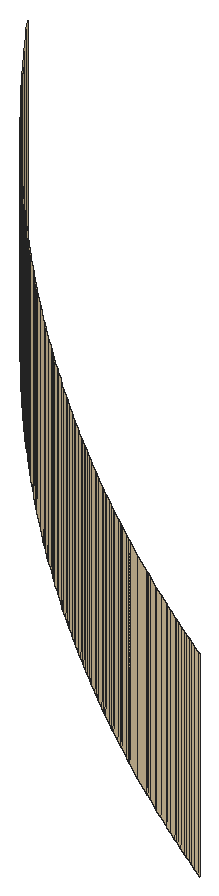
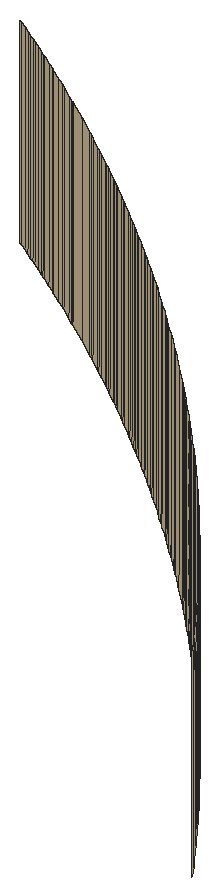
# SketchUp Ruby script. Lengths in inches.
U = 1.inch
M = Sketchup.active_model
def pt(a) = Geom::Point3d.new(a.map { |v| v * U })
def face(e, loops, mat)
  f = e.add_face(loops[0].map { |a| pt(a) })
  loops[1..].each { |l| e.add_face(l.map { |a| pt(a) }).erase! }
  f.material = f.back_material = mat if mat
  f
end
# faces: each face lists its corners as indices into pts; further lists are holes
def faces(e, pts, list, mat = nil) = list.each { |f| face(e, (f[0].is_a?(Array) ? f : [f]).map { |l| l.map { |i| pts[i] } }, mat) }
# xy, xz, yz: faces in a plane at the given z, y or x. An outline is a flat list of corners, or four numbers for a rectangle; further outlines are holes
def ring(l) = l.size == 4 ? [[l[0], l[1]], [l[2], l[1]], [l[2], l[3]], [l[0], l[3]]] : l.each_slice(2).to_a
def flat(e, list, mat, &to3) = list.each { |f| face(e, (f[0].is_a?(Array) ? f : [f]).map { |l| ring(l).map { |u, v| to3.(u, v) } }, mat) }
def xy(e, z, list, mat = nil) = flat(e, list, mat) { |x, y| [x, y, z] }
def xz(e, y, list, mat = nil) = flat(e, list, mat) { |x, z| [x, y, z] }
def yz(e, x, list, mat = nil) = flat(e, list, mat) { |y, z| [x, y, z] }
def lines(e, pts, list) = list.each { |a, b| e.add_line(pt(pts[a]), pt(pts[b])) }
# prism: a flat outline (further loops are holes) pulled along v
def prism(e, loops, v, mat = nil)
  f = face(e, loops, mat); d = Geom::Vector3d.new(v.map { |x| x * U })
  f.pushpull(f.normal.samedirection?(d) ? d.length : -d.length)
end
def box(e, o, s, mat = nil) = prism(e, [[o, [o[0] + s[0], o[1], o[2]], [o[0] + s[0], o[1] + s[1], o[2]], [o[0], o[1] + s[1], o[2]]]], [0, 0, s[2]], mat)
def at(x, y, z, deg = 0) = Geom::Transformation.translation(pt([x, y, z])) * Geom::Transformation.rotation(ORIGIN, Z_AXIS, deg.degrees)
def axes(o, x, y, z) = Geom::Transformation.new([*x, 0, *y, 0, *z, 0, *pt(o).to_a, 1])
def part(name) = M.definitions.add(name)
# library, detail: a bought-in or finely detailed component or shape, given as its bounding box
def library(name, o, s) = part(name).tap { |d| box(d.entities, o, s) }
def detail(e, o, s) = box(e.add_group.entities, o, s)
def put(e, d, t, mat = nil) = e.add_instance(d, t).tap { |i| i.material = mat if mat }
def group(e, t, mat = nil) = e.add_group.tap { |g| g.transformation = t; g.material = mat if mat }.entities
root = M.entities
M.materials.add("1026 AP 7946 SUNNY SIDE UP").color = [254, 231, 186]
p = [[16.068,217.047,276],[16.027,217.074,276],[16.027,217.074,274],[16.068,217.047,274],[15.982,217.102,276],[15.905,217.152,276],
  [15.905,217.152,274],[15.982,217.102,274],[15.768,217.241,276],[15.682,217.298,276],[15.682,217.298,274],[15.768,217.241,274],
  [15.805,217.217,276],[15.805,217.217,274],[15.839,217.195,276],[15.839,217.195,274],[15.612,217.344,276],[15.584,217.362,276],
  [15.584,217.362,274],[15.612,217.344,274],[15.46,217.446,276],[15.386,217.496,276],[15.386,217.496,274],[15.46,217.446,274],
  [15.555,217.382,276],[15.555,217.382,274],[15.344,217.525,276],[15.236,217.599,276],[15.236,217.599,274],[15.344,217.525,274],
  [15.365,217.51,276],[15.365,217.51,274],[15.161,217.65,276],[15.161,217.65,274],[15.133,217.67,276],[15.006,217.759,276],
  [15.006,217.759,274],[15.133,217.67,274],[15.148,217.66,276],[15.148,217.66,274],[14.925,217.817,276],[14.718,217.966,276],
  [14.718,217.966,274],[14.925,217.817,274],[14.932,217.812,276],[14.932,217.812,274],[14.939,217.807,276],[14.939,217.807,274],
  [14.512,218.117,276],[14.512,218.117,274],[14.498,218.127,276],[14.432,218.176,276],[14.432,218.176,274],[14.498,218.127,274],
  [14.505,218.122,276],[14.505,218.122,274],[14.308,218.27,276],[14.308,218.27,274],[14.209,218.345,276],[14.105,218.425,276],
  [14.105,218.425,274],[14.209,218.345,274],[14.28,218.29,276],[14.28,218.29,274],[14.294,218.28,276],[14.294,218.28,274],
  [14.084,218.441,276],[14.064,218.456,276],[14.064,218.456,274],[14.084,218.441,274],[13.994,218.511,276],[13.904,218.582,276],
  [13.904,218.582,274],[13.994,218.511,274],[13.85,218.624,276],[13.784,218.677,276],[13.784,218.677,274],[13.85,218.624,274],
  [13.876,218.604,276],[13.876,218.604,274],[13.704,218.741,276],[13.67,218.769,276],[13.67,218.769,274],[13.704,218.741,274],
  [13.577,218.844,276],[13.506,218.902,276],[13.506,218.902,274],[13.577,218.844,274],[13.638,218.794,276],[13.638,218.794,274],
  [13.465,218.936,276],[13.427,218.967,276],[13.427,218.967,274],[13.465,218.936,274],[13.372,219.012,276],[13.309,219.065,276],
  [13.309,219.065,274],[13.372,219.012,274],[13.218,219.141,276],[13.169,219.183,276],[13.169,219.183,274],[13.218,219.141,274],
  [13.262,219.105,276],[13.262,219.105,274],[13.114,219.229,276],[13.06,219.276,276],[13.06,219.276,274],[13.114,219.229,274],
  [13.011,219.318,276],[12.968,219.355,276],[12.968,219.355,274],[13.011,219.318,274],[12.921,219.396,276],[12.86,219.45,276],
  [12.86,219.45,274],[12.921,219.396,274],[12.769,219.53,276],[12.729,219.565,276],[12.729,219.565,274],[12.769,219.53,274],
  [12.806,219.497,276],[12.806,219.497,274],[12.661,219.626,276],[12.603,219.678,276],[12.603,219.678,274],[12.661,219.626,274],
  [12.539,219.735,276],[12.464,219.805,276],[12.464,219.805,274],[12.539,219.735,274],[12.572,219.706,276],[12.572,219.706,274],
  [12.401,219.861,276],[12.401,219.861,274],[12.351,219.908,276],[12.267,219.986,276],[12.267,219.986,274],[12.351,219.908,274],
  [12.377,219.884,276],[12.377,219.884,274],[12.202,220.047,276],[12.184,220.064,276],[12.184,220.064,274],[12.202,220.047,274],
  [12.165,220.082,276],[12.07,220.172,276],[12.07,220.172,274],[12.165,220.082,274],[11.992,220.246,276],[11.98,220.258,276],
  [11.98,220.258,274],[11.992,220.246,274],[12.004,220.234,276],[12.004,220.234,274],[11.868,220.366,276],[11.868,220.366,274],
  [11.797,220.436,276],[11.615,220.615,276],[11.615,220.615,274],[11.797,220.436,274],[11.803,220.43,276],[11.803,220.43,274],
  [11.809,220.424,276],[11.809,220.424,274],[11.436,220.797,276],[11.436,220.797,274],[11.424,220.809,276],[11.366,220.868,276],
  [11.366,220.868,274],[11.424,220.809,274],[11.43,220.803,276],[11.43,220.803,274],[11.258,220.98,276],[11.258,220.98,274],
  [11.234,221.004,276],[11.172,221.07,276],[11.172,221.07,274],[11.234,221.004,274],[11.246,220.992,276],[11.246,220.992,274],
  [11.082,221.165,276],[11.082,221.165,274],[11.047,221.202,276],[10.986,221.267,276],[10.986,221.267,274],[11.047,221.202,274],
  [11.064,221.184,276],[11.064,221.184,274],[10.908,221.351,276],[10.908,221.351,274],[10.861,221.401,276],[10.805,221.464,276],
  [10.805,221.464,274],[10.861,221.401,274],[10.884,221.377,276],[10.884,221.377,274],[10.735,221.539,276],[10.706,221.572,276],
  [10.706,221.572,274],[10.735,221.539,274],[10.678,221.603,276],[10.626,221.661,276],[10.626,221.661,274],[10.678,221.603,274],
  [10.565,221.729,276],[10.53,221.769,276],[10.53,221.769,274],[10.565,221.729,274],[10.497,221.806,276],[10.45,221.86,276],
  [10.45,221.86,274],[10.497,221.806,274],[10.396,221.921,276],[10.355,221.968,276],[10.355,221.968,274],[10.396,221.921,274],
  [10.318,222.011,276],[10.276,222.06,276],[10.276,222.06,274],[10.318,222.011,274],[10.229,222.114,276],[10.183,222.169,276],
  [10.183,222.169,274],[10.229,222.114,274],[10.141,222.218,276],[10.105,222.262,276],[10.105,222.262,274],[10.141,222.218,274],
  [10.065,222.309,276],[10.012,222.372,276],[10.012,222.372,274],[10.065,222.309,274],[9.967,222.427,276],[9.936,222.465,276],
  [9.936,222.465,274],[9.967,222.427,274],[9.902,222.506,276],[9.844,222.577,276],[9.844,222.577,274],[9.902,222.506,274],
  [9.794,222.638,276],[9.769,222.67,276],[9.769,222.67,274],[9.794,222.638,274],[9.741,222.704,276],[9.677,222.784,276],
  [9.677,222.784,274],[9.741,222.704,274],[9.624,222.85,276],[9.624,222.85,274],[9.582,222.904,276],[9.511,222.994,276],
  [9.511,222.994,274],[9.582,222.904,274],[9.604,222.876,276],[9.604,222.876,274],[9.456,223.064,276],[9.456,223.064,274],
  [9.425,223.105,276],[9.345,223.209,276],[9.345,223.209,274],[9.425,223.105,274],[9.441,223.084,276],[9.441,223.084,274],
  [9.29,223.28,276],[9.29,223.28,274],[9.27,223.308,276],[9.176,223.432,276],[9.176,223.432,274],[9.27,223.308,274],
  [9.28,223.294,276],[9.28,223.294,274],[9.127,223.498,276],[9.127,223.498,274],[9.117,223.512,276],[8.966,223.718,276],
  [8.966,223.718,274],[9.117,223.512,274],[9.122,223.505,276],[9.122,223.505,274],[8.817,223.925,276],[8.817,223.925,274],
  [8.807,223.939,276],[8.759,224.006,276],[8.759,224.006,274],[8.807,223.939,274],[8.812,223.932,276],[8.812,223.932,274],
  [8.67,224.133,276],[8.67,224.133,274]]
faces(root,p,[[0,1,2,3],[4,5,6,7],[1,4,7,2],[8,9,10,11],[12,8,11,13],[14,12,13,15],[5,14,15,6],[16,17,18,19],
  [9,16,19,10],[20,21,22,23],[24,20,23,25],[17,24,25,18],[26,27,28,29],[30,26,29,31],[21,30,31,22],[27,32,33,28],
  [34,35,36,37],[38,34,37,39],[32,38,39,33],[40,41,42,43],[44,40,43,45],[46,44,45,47],[35,46,47,36],[41,48,49,42],
  [50,51,52,53],[54,50,53,55],[48,54,55,49],[51,56,57,52],[58,59,60,61],[62,58,61,63],[64,62,63,65],[56,64,65,57],
  [66,67,68,69],[59,66,69,60],[70,71,72,73],[67,70,73,68],[74,75,76,77],[78,74,77,79],[71,78,79,72],[80,81,82,83],
  [75,80,83,76],[84,85,86,87],[88,84,87,89],[81,88,89,82],[90,91,92,93],[85,90,93,86],[94,95,96,97],[91,94,97,92],
  [98,99,100,101],[102,98,101,103],[95,102,103,96],[104,105,106,107],[99,104,107,100],[108,109,110,111],[105,108,111,106],[112,113,114,115],
  [109,112,115,110],[116,117,118,119],[120,116,119,121],[113,120,121,114],[122,123,124,125],[117,122,125,118],[126,127,128,129],[130,126,129,131],
  [123,130,131,124],[127,132,133,128],[134,135,136,137],[138,134,137,139],[132,138,139,133],[140,141,142,143],[135,140,143,136],[144,145,146,147],
  [141,144,147,142],[148,149,150,151],[152,148,151,153],[145,152,153,146],[149,154,155,150],[156,157,158,159],[160,156,159,161],[162,160,161,163],
  [154,162,163,155],[157,164,165,158],[166,167,168,169],[170,166,169,171],[164,170,171,165],[167,172,173,168],[174,175,176,177],[178,174,177,179],
  [172,178,179,173],[175,180,181,176],[182,183,184,185],[186,182,185,187],[180,186,187,181],[183,188,189,184],[190,191,192,193],[194,190,193,195],
  [188,194,195,189],[196,197,198,199],[191,196,199,192],[200,201,202,203],[197,200,203,198],[204,205,206,207],[201,204,207,202],[208,209,210,211],
  [205,208,211,206],[212,213,214,215],[209,212,215,210],[216,217,218,219],[213,216,219,214],[220,221,222,223],[217,220,223,218],[224,225,226,227],
  [221,224,227,222],[228,229,230,231],[225,228,231,226],[232,233,234,235],[229,232,235,230],[236,237,238,239],[233,236,239,234],[240,241,242,243],
  [237,240,243,238],[244,245,246,247],[241,244,247,242],[245,248,249,246],[250,251,252,253],[254,250,253,255],[248,254,255,249],[251,256,257,252],
  [258,259,260,261],[262,258,261,263],[256,262,263,257],[259,264,265,260],[266,267,268,269],[270,266,269,271],[264,270,271,265],[267,272,273,268],
  [274,275,276,277],[278,274,277,279],[272,278,279,273],[275,280,281,276],[282,283,284,285],[286,282,285,287],[280,286,287,281],[283,288,289,284]],"1026 AP 7946 SUNNY SIDE UP")
